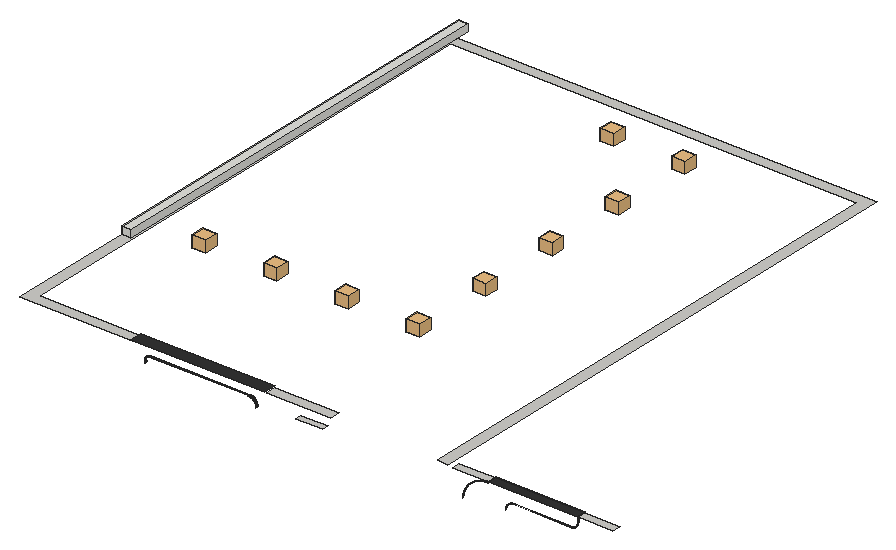
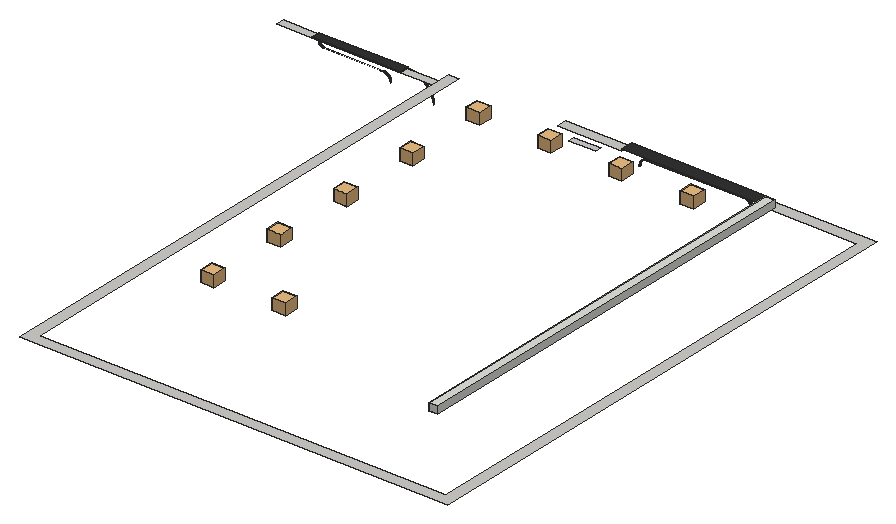
# SketchUp Ruby script. Lengths in inches.
U = 1.inch
M = Sketchup.active_model
def pt(a) = Geom::Point3d.new(a.map { |v| v * U })
def face(e, loops, mat)
  f = e.add_face(loops[0].map { |a| pt(a) })
  loops[1..].each { |l| e.add_face(l.map { |a| pt(a) }).erase! }
  f.material = f.back_material = mat if mat
  f
end
# faces: each face lists its corners as indices into pts; further lists are holes
def faces(e, pts, list, mat = nil) = list.each { |f| face(e, (f[0].is_a?(Array) ? f : [f]).map { |l| l.map { |i| pts[i] } }, mat) }
# xy, xz, yz: faces in a plane at the given z, y or x. An outline is a flat list of corners, or four numbers for a rectangle; further outlines are holes
def ring(l) = l.size == 4 ? [[l[0], l[1]], [l[2], l[1]], [l[2], l[3]], [l[0], l[3]]] : l.each_slice(2).to_a
def flat(e, list, mat, &to3) = list.each { |f| face(e, (f[0].is_a?(Array) ? f : [f]).map { |l| ring(l).map { |u, v| to3.(u, v) } }, mat) }
def xy(e, z, list, mat = nil) = flat(e, list, mat) { |x, y| [x, y, z] }
def xz(e, y, list, mat = nil) = flat(e, list, mat) { |x, z| [x, y, z] }
def yz(e, x, list, mat = nil) = flat(e, list, mat) { |y, z| [x, y, z] }
def lines(e, pts, list) = list.each { |a, b| e.add_line(pt(pts[a]), pt(pts[b])) }
# prism: a flat outline (further loops are holes) pulled along v
def prism(e, loops, v, mat = nil)
  f = face(e, loops, mat); d = Geom::Vector3d.new(v.map { |x| x * U })
  f.pushpull(f.normal.samedirection?(d) ? d.length : -d.length)
end
def box(e, o, s, mat = nil) = prism(e, [[o, [o[0] + s[0], o[1], o[2]], [o[0] + s[0], o[1] + s[1], o[2]], [o[0], o[1] + s[1], o[2]]]], [0, 0, s[2]], mat)
def at(x, y, z, deg = 0) = Geom::Transformation.translation(pt([x, y, z])) * Geom::Transformation.rotation(ORIGIN, Z_AXIS, deg.degrees)
def axes(o, x, y, z) = Geom::Transformation.new([*x, 0, *y, 0, *z, 0, *pt(o).to_a, 1])
def part(name) = M.definitions.add(name)
# library, detail: a bought-in or finely detailed component or shape, given as its bounding box
def library(name, o, s) = part(name).tap { |d| box(d.entities, o, s) }
def detail(e, o, s) = box(e.add_group.entities, o, s)
def put(e, d, t, mat = nil) = e.add_instance(d, t).tap { |i| i.material = mat if mat }
def group(e, t, mat = nil) = e.add_group.tap { |g| g.transformation = t; g.material = mat if mat }.entities
root = M.entities
M.materials.add("[Granite Dark Gray]").color = [51, 50, 50]
M.materials.add("[Stone Sandstone Ashlar Light]").color = [206, 205, 201]
c1 = library("6",[-5.64,-5.64,-12.71],[15.28,15.28,12.71])
xy(root,52.99,[[548.53,53,548.6875,54]],"[Granite Dark Gray]")
xy(root,53,[[548.84,53,549,54],[549,53,615,54],[615,53,615.12,54],[615.12,53,615.24,54]],"[Granite Dark Gray]")
xy(root,57,[[309,48,339,55]],"[Stone Sandstone Ashlar Light]")
xy(root,62.99,[[257.3125,46,257.47,48]],"[Granite Dark Gray]")
xy(root,63,[[146,46,257,48],[257,46,257.16,48]],"[Granite Dark Gray]")
xy(root,65,[[520.54,53,521,54]],"[Granite Dark Gray]")
xy(root,65,[[480,54,521,63],[621,54,660,63]],"[Stone Sandstone Ashlar Light]")
xy(root,66,[[521,53,621,63]],"[Granite Dark Gray]")
xy(root,71,[[0,48,126,48,126,60,12,60,12,636,468,636,468,48,480,48,480,648,0,648],[276,48,348,60]],"[Stone Sandstone Ashlar Light]")
xy(root,73,[[126,46,276,60]],"[Granite Dark Gray]")
xz(root,63,[[521,65,621,66]],"[Granite Dark Gray]")
yz(root,141.17,[[46,57.16,48,57.29],[46,57.29,48,57.42],[46,57.42,48,57.56]],"[Granite Dark Gray]")
yz(root,265.99,[[46,54.3125,48,54.47]],"[Granite Dark Gray]")
yz(root,266,[[46,54,48,54.16]],"[Granite Dark Gray]")
yz(root,521,[[53,65,63,66]],"[Granite Dark Gray]")
yz(root,540,[[53,44,54,44.16]],"[Granite Dark Gray]")
yz(root,540.01,[[53,44.3125,54,44.47]],"[Granite Dark Gray]")
yz(root,621,[[53,58.76,54,58.88],[53,58.88,54,59],[53,59,54,59,54,65,63,65,63,66,53,66]],"[Granite Dark Gray]")
p = [[491.79,54,39.66],[491.73,54,39.2],[491.73,53,39.2],[491.79,53,39.66],[491.86,54,40.11],[491.86,53,40.11],
  [491.9375,54,40.57],[491.9375,53,40.57],[492.02,54,41.03],[492.02,53,41.03],[492.11,54,41.48],[492.11,53,41.48],
  [492.21,54,41.94],[492.21,53,41.94],[492.32,54,42.39],[492.32,53,42.39],[492.43,54,42.84],[492.43,53,42.84],
  [492.55,54,43.28],[492.55,53,43.28],[492.67,54,43.73],[492.67,53,43.73],[492.8,54,44.17],[492.8,53,44.17],
  [492.94,54,44.62],[492.94,53,44.62],[540,54,44.16],[540.01,54,44.3125],[540.01,53,44.3125],[540,53,44.16],
  [540.01,54,44.47],[540.02,54,44.63],[540.02,53,44.63],[540.01,53,44.47],[493.09,54,45.06],[493.09,53,45.06],
  [540.03,54,44.78],[540.03,53,44.78],[540.05,54,44.94],[540.05,53,44.94],[540.07,54,45.1],[540.07,53,45.1],
  [493.24,54,45.49],[493.24,53,45.49],[540.09,54,45.25],[540.09,53,45.25],[540.11,54,45.41],[540.11,53,45.41],
  [540.14,54,45.5625],[540.14,53,45.5625],[493.4,54,45.93],[493.4,53,45.93],[540.17,54,45.72],[540.17,53,45.72],
  [540.2,54,45.87],[540.2,53,45.87],[493.57,54,46.36],[493.57,53,46.36],[540.23,54,46.02],[540.23,53,46.02],
  [540.27,54,46.18],[540.27,53,46.18],[540.31,54,46.33],[540.31,53,46.33],[540.35,54,46.48],[540.35,53,46.48],
  [493.75,54,46.79],[493.75,53,46.79],[540.39,54,46.63],[540.39,53,46.63],[540.44,54,46.78],[540.44,53,46.78],
  [493.93,54,47.22],[493.93,53,47.22],[540.49,54,46.93],[540.49,53,46.93],[540.54,54,47.08],[540.54,53,47.08],
  [540.6,54,47.23],[540.6,53,47.23],[494.11,54,47.64],[494.11,53,47.64],[540.66,54,47.37],[540.66,53,47.37],
  [540.72,54,47.52],[540.72,53,47.52],[540.78,54,47.66],[540.78,53,47.66],[494.31,54,48.06],[494.31,53,48.06],
  [540.84,54,47.8],[540.84,53,47.8],[540.91,54,47.95],[540.91,53,47.95],[540.98,54,48.09],[540.98,53,48.09],
  [494.51,54,48.48],[494.51,53,48.48],[541.05,54,48.23],[541.05,53,48.23],[541.13,54,48.36],[541.13,53,48.36],
  [541.21,54,48.5],[541.21,53,48.5],[494.72,54,48.89],[494.72,53,48.89],[541.29,54,48.64],[541.29,53,48.64],
  [541.37,54,48.77],[541.37,53,48.77],[541.45,54,48.9],[541.45,53,48.9],[494.93,54,49.3],[494.93,53,49.3],
  [541.54,54,49.03],[541.54,53,49.03],[541.63,54,49.16],[541.63,53,49.16],[541.72,54,49.29],[541.72,53,49.29],
  [495.15,54,49.71],[495.15,53,49.71],[541.8125,54,49.42],[541.8125,53,49.42],[541.91,54,49.54],[541.91,53,49.54],
  [542.01,54,49.66],[542.01,53,49.66],[495.375,54,50.12],[495.375,53,50.12],[542.11,54,49.79],[542.11,53,49.79],
  [542.21,54,49.9],[542.21,53,49.9],[542.3125,54,50.02],[542.3125,53,50.02],[542.42,54,50.14],[542.42,53,50.14],
  [495.61,54,50.52],[495.61,53,50.52],[542.53,54,50.25],[542.53,53,50.25],[542.64,54,50.36],[542.64,53,50.36],
  [542.75,54,50.47],[542.75,53,50.47],[495.85,54,50.91],[495.85,53,50.91],[542.86,54,50.58],[542.86,53,50.58],
  [542.98,54,50.6875],[542.98,53,50.6875],[543.1,54,50.79],[543.1,53,50.79],[543.21,54,50.89],[543.21,53,50.89],
  [496.09,54,51.31],[496.09,53,51.31],[543.34,54,50.99],[543.34,53,50.99],[543.46,54,51.09],[543.46,53,51.09],
  [543.58,54,51.1875],[543.58,53,51.1875],[543.71,54,51.28],[543.71,53,51.28],[496.34,54,51.7],[496.34,53,51.7],
  [543.84,54,51.37],[543.84,53,51.37],[543.97,54,51.46],[543.97,53,51.46],[544.1,54,51.55],[544.1,53,51.55],
  [544.23,54,51.63],[544.23,53,51.63],[544.36,54,51.71],[544.36,53,51.71],[496.6,54,52.08],[496.6,53,52.08],
  [544.5,54,51.79],[544.5,53,51.79],[544.64,54,51.87],[544.64,53,51.87],[544.77,54,51.95],[544.77,53,51.95],
  [544.91,54,52.02],[544.91,53,52.02],[545.05,54,52.09],[545.05,53,52.09],[496.86,54,52.46],[496.86,53,52.46],
  [545.2,54,52.16],[545.2,53,52.16],[545.34,54,52.22],[545.34,53,52.22],[545.48,54,52.28],[545.48,53,52.28],
  [545.63,54,52.34],[545.63,53,52.34],[545.77,54,52.4],[545.77,53,52.4],[545.92,54,52.46],[545.92,53,52.46],
  [497.13,54,52.84],[497.13,53,52.84],[546.07,54,52.51],[546.07,53,52.51],[546.22,54,52.56],[546.22,53,52.56],
  [546.37,54,52.61],[546.37,53,52.61],[546.52,54,52.65],[546.52,53,52.65],[546.67,54,52.69],[546.67,53,52.69],
  [546.82,54,52.73],[546.82,53,52.73],[546.98,54,52.77],[546.98,53,52.77],[497.41,54,53.21],[497.41,53,53.21],
  [547.13,54,52.8],[547.13,53,52.8],[547.28,54,52.83],[547.28,53,52.83],[547.4375,54,52.86],[547.4375,53,52.86],
  [547.59,54,52.89],[547.59,53,52.89],[547.75,54,52.91],[547.75,53,52.91],[547.9,54,52.93],[547.9,53,52.93],
  [548.06,54,52.95],[548.06,53,52.95],[548.22,54,52.97],[548.22,53,52.97],[548.37,54,52.98],[548.37,53,52.98],
  [548.53,54,52.99],[548.53,53,52.99],[548.6875,54,52.99],[548.84,54,53],[548.84,53,53],[548.6875,53,52.99],
  [615.24,54,53],[615.35,54,53.01],[615.35,53,53.01],[615.24,53,53],[615.47,54,53.02],[615.47,53,53.02],
  [615.59,54,53.03],[615.59,53,53.03],[615.71,54,53.04],[615.71,53,53.04],[615.82,54,53.06],[615.82,53,53.06],
  [615.9375,54,53.07],[615.9375,53,53.07],[616.05,54,53.09],[616.05,53,53.09],[616.17,54,53.12],[616.17,53,53.12],
  [616.29,54,53.14],[616.29,53,53.14],[616.4,54,53.17],[616.4,53,53.17],[497.69,54,53.58],[497.69,53,53.58],
  [616.51,54,53.19],[616.51,53,53.19],[616.63,54,53.23],[616.63,53,53.23],[616.74,54,53.26],[616.74,53,53.26],
  [616.85,54,53.29],[616.85,53,53.29],[616.97,54,53.33],[616.97,53,53.33],[617.08,54,53.37],[617.08,53,53.37],
  [617.1875,54,53.41],[617.1875,53,53.41],[617.3,54,53.46],[617.3,53,53.46],[617.4,54,53.5],[617.4,53,53.5],
  [617.51,54,53.55],[617.51,53,53.55],[497.98,54,53.94],[497.98,53,53.94],[617.62,54,53.6],[617.62,53,53.6],
  [617.72,54,53.65],[617.72,53,53.65],[617.83,54,53.71],[617.83,53,53.71],[617.93,54,53.77],[617.93,53,53.77],
  [618.03,54,53.82],[618.03,53,53.82],[618.13,54,53.88],[618.13,53,53.88],[498.27,54,54.3],[498.27,53,54.3],
  [618.23,54,53.95],[618.23,53,53.95],[618.33,54,54.01],[618.33,53,54.01],[618.43,54,54.08],[618.43,53,54.08],
  [618.53,54,54.15],[618.53,53,54.15],[618.62,54,54.22],[618.62,53,54.22],[266,46,54.16],[265.99,46,54.3125],
  [265.99,48,54.3125],[266,48,54.16],[618.71,54,54.29],[618.71,53,54.29],[498.57,54,54.66],[498.57,53,54.66],
  [618.81,54,54.36],[618.81,53,54.36],[618.9,54,54.4375],[618.9,53,54.4375],[618.99,54,54.51],[618.99,53,54.51],
  [265.99,46,54.47],[265.98,46,54.63],[265.98,48,54.63],[265.99,48,54.47],[619.07,54,54.59],[619.07,53,54.59],
  [265.97,46,54.78],[265.97,48,54.78],[619.16,54,54.67],[619.16,53,54.67],[498.87,54,55.01],[498.87,53,55.01],
  [619.24,54,54.76],[619.24,53,54.76],[265.95,46,54.94],[265.95,48,54.94],[619.33,54,54.84],[619.33,53,54.84],
  [619.41,54,54.93],[619.41,53,54.93],[265.93,46,55.1],[265.93,48,55.1],[619.49,54,55.01],[619.49,53,55.01],
  [141.64,46,55.12],[141.69,46,55],[141.69,48,55],[141.64,48,55.12],[499.18,54,55.35],[499.18,53,55.35],
  [619.5625,54,55.1],[619.5625,53,55.1],[141.59,46,55.24],[141.59,48,55.24],[265.91,46,55.25],[265.91,48,55.25],
  [619.64,54,55.19],[619.64,53,55.19],[141.54,46,55.36],[141.54,48,55.36],[619.71,54,55.29],[619.71,53,55.29],
  [265.89,46,55.41],[265.89,48,55.41],[619.78,54,55.38],[619.78,53,55.38],[141.49,46,55.49],[141.49,48,55.49],
  [265.86,46,55.5625],[265.86,48,55.5625],[499.5,54,55.69],[499.5,53,55.69],[619.85,54,55.47],[619.85,53,55.47],
  [141.45,46,55.61],[141.45,48,55.61],[619.92,54,55.57],[619.92,53,55.57],[141.41,46,55.74],[141.41,48,55.74],
  [265.83,46,55.72],[265.83,48,55.72],[619.99,54,55.67],[619.99,53,55.67],[141.375,46,55.86],[141.375,48,55.86],
  [265.8,46,55.87],[265.8,48,55.87],[499.82,54,56.03],[499.82,53,56.03],[620.05,54,55.77],[620.05,53,55.77],
  [620.12,54,55.87],[620.12,53,55.87],[141.34,46,55.99],[141.34,48,55.99],[265.77,46,56.02],[265.77,48,56.02],
  [620.18,54,55.97],[620.18,53,55.97],[141.3125,46,56.12],[141.3125,48,56.12],[265.73,46,56.18],[265.73,48,56.18],
  [500.14,54,56.36],[500.14,53,56.36],[620.23,54,56.07],[620.23,53,56.07],[141.28,46,56.25],[141.28,48,56.25],
  [620.29,54,56.17],[620.29,53,56.17],[141.26,46,56.38],[141.26,48,56.38],[265.69,46,56.33],[265.69,48,56.33],
  [620.35,54,56.28],[620.35,53,56.28],[265.65,46,56.48],[265.65,48,56.48],[620.4,54,56.38],[620.4,53,56.38],
  [141.24,46,56.51],[141.24,48,56.51],[500.47,54,56.68],[500.47,53,56.68],[620.45,54,56.49],[620.45,53,56.49],
  [141.22,46,56.64],[141.22,48,56.64],[265.61,46,56.63],[265.61,48,56.63],[620.5,54,56.6],[620.5,53,56.6],
  [141.2,46,56.77],[141.2,48,56.77],[265.56,46,56.78],[265.56,48,56.78],[620.54,54,56.7],[620.54,53,56.7],
  [500.81,54,57],[500.81,53,57],[620.59,54,56.8125],[620.59,53,56.8125],[141.19,46,56.9],[141.19,48,56.9],
  [265.51,46,56.93],[265.51,48,56.93],[620.63,54,56.92],[620.63,53,56.92],[141.18,46,57.03],[141.18,48,57.03],
  [265.46,46,57.08],[265.46,48,57.08],[620.67,54,57.03],[620.67,53,57.03],[141.17,46,57.16],[141.17,48,57.16],
  [501.15,54,57.32],[501.15,53,57.32],[620.71,54,57.15],[620.71,53,57.15],[265.4,46,57.23],[265.4,48,57.23],
  [620.74,54,57.26],[620.74,53,57.26],[265.34,46,57.37],[265.34,48,57.37],[501.49,54,57.63],[501.49,53,57.63],
  [620.77,54,57.37],[620.77,53,57.37],[265.28,46,57.52],[265.28,48,57.52],[620.81,54,57.49],[620.81,53,57.49],
  [265.22,46,57.66],[265.22,48,57.66],[620.83,54,57.6],[620.83,53,57.6],[141.18,46,57.6875],[141.17,46,57.56],
  [141.17,48,57.56],[141.18,48,57.6875],[501.84,54,57.93],[501.84,53,57.93],[620.86,54,57.71],[620.86,53,57.71],
  [141.1875,46,57.82],[141.1875,48,57.82],[265.16,46,57.8],[265.16,48,57.8],[620.88,54,57.83],[620.88,53,57.83],
  [141.2,46,57.95],[141.2,48,57.95],[265.09,46,57.95],[265.09,48,57.95],[620.91,54,57.95],[620.91,53,57.95],
  [265.02,46,58.09],[265.02,48,58.09],[502.2,54,58.23],[502.2,53,58.23],[620.93,54,58.0625],[620.93,53,58.0625],
  [141.21,46,58.08],[141.21,48,58.08],[141.23,46,58.21],[141.23,48,58.21],[264.95,46,58.23],[264.95,48,58.23],
  [620.94,54,58.18],[620.94,53,58.18],[141.25,46,58.34],[141.25,48,58.34],[264.87,46,58.36],[264.87,48,58.36],
  [502.56,54,58.52],[502.56,53,58.52],[620.96,54,58.29],[620.96,53,58.29],[141.27,46,58.47],[141.27,48,58.47],
  [620.97,54,58.41],[620.97,53,58.41],[264.79,46,58.5],[264.79,48,58.5],[620.98,54,58.53],[620.98,53,58.53],
  [141.3,46,58.6],[141.3,48,58.6],[264.71,46,58.64],[264.71,48,58.64],[502.92,54,58.81],[502.92,53,58.81],
  [620.99,54,58.65],[620.99,53,58.65],[141.33,46,58.73],[141.33,48,58.73],[264.63,46,58.77],[264.63,48,58.77],
  [621,54,58.76],[621,53,58.76],[141.36,46,58.86],[141.36,48,58.86],[264.55,46,58.9],[264.55,48,58.9],
  [503.29,54,59.09],[503.29,53,59.09],[141.4,46,58.98],[141.4,48,58.98],[264.46,46,59.03],[264.46,48,59.03],
  [141.4375,46,59.11],[141.4375,48,59.11],[264.37,46,59.16],[264.37,48,59.16],[141.48,46,59.23],[141.48,48,59.23],
  [503.66,54,59.37],[503.66,53,59.37],[141.52,46,59.36],[141.52,48,59.36],[264.28,46,59.29],[264.28,48,59.29],
  [264.1875,46,59.42],[264.1875,48,59.42],[141.57,46,59.48],[141.57,48,59.48],[264.09,46,59.54],[264.09,48,59.54],
  [504.04,54,59.64],[504.04,53,59.64],[141.62,46,59.6],[141.62,48,59.6],[263.99,46,59.66],[263.99,48,59.66],
  [141.67,46,59.72],[141.67,48,59.72],[504.42,54,59.9],[504.42,53,59.9],[141.73,46,59.84],[141.73,48,59.84],
  [263.89,46,59.79],[263.89,48,59.79],[141.79,46,59.96],[141.79,48,59.96],[263.79,46,59.9],[263.79,48,59.9],
  [263.6875,46,60.02],[263.6875,48,60.02],[504.8,54,60.16],[504.8,53,60.16],[141.85,46,60.08],[141.85,48,60.08],
  [263.58,46,60.14],[263.58,48,60.14],[141.91,46,60.19],[141.91,48,60.19],[263.47,46,60.25],[263.47,48,60.25],
  [141.98,46,60.3],[141.98,48,60.3],[505.19,54,60.41],[505.19,53,60.41],[142.05,46,60.42],[142.05,48,60.42],
  [263.36,46,60.36],[263.36,48,60.36],[142.12,46,60.53],[142.12,48,60.53],[263.25,46,60.47],[263.25,48,60.47],
  [505.59,54,60.65],[505.59,53,60.65],[142.19,46,60.64],[142.19,48,60.64],[263.14,46,60.58],[263.14,48,60.58],
  [142.27,46,60.74],[142.27,48,60.74],[263.02,46,60.6875],[263.02,48,60.6875],[142.35,46,60.85],[142.35,48,60.85],
  [262.9,46,60.79],[262.9,48,60.79],[505.98,54,60.89],[505.98,53,60.89],[142.43,46,60.95],[142.43,48,60.95],
  [262.79,46,60.89],[262.79,48,60.89],[262.66,46,60.99],[262.66,48,60.99],[506.38,54,61.125],[506.38,53,61.125],
  [142.51,46,61.05],[142.51,48,61.05],[262.54,46,61.09],[262.54,48,61.09],[142.6,46,61.15],[142.6,48,61.15],
  [262.42,46,61.1875],[262.42,48,61.1875],[506.79,54,61.35],[506.79,53,61.35],[142.6875,46,61.25],[142.6875,48,61.25],
  [142.78,46,61.34],[142.78,48,61.34],[262.29,46,61.28],[262.29,48,61.28],[142.87,46,61.4375],[142.87,48,61.4375],
  [262.16,46,61.37],[262.16,48,61.37],[142.97,46,61.53],[142.97,48,61.53],[262.03,46,61.46],[262.03,48,61.46],
  [507.2,54,61.57],[507.2,53,61.57],[143.06,46,61.62],[143.06,48,61.62],[261.9,46,61.55],[261.77,46,61.63],
  [261.77,48,61.63],[261.9,48,61.55],[143.16,46,61.7],[143.16,48,61.7],[261.64,46,61.71],[261.64,48,61.71],
  [507.61,54,61.78],[507.61,53,61.78],[143.26,46,61.79],[143.26,48,61.79],[261.5,46,61.79],[261.5,48,61.79],
  [143.37,46,61.87],[143.37,48,61.87],[261.36,46,61.87],[261.36,48,61.87],[508.02,54,61.99],[508.02,53,61.99],
  [143.47,46,61.95],[143.47,48,61.95],[261.23,46,61.95],[261.09,46,62.02],[261.09,48,62.02],[261.23,48,61.95],
  [143.58,46,62.03],[143.58,48,62.03],[143.6875,46,62.1],[143.6875,48,62.1],[260.95,46,62.09],[260.95,48,62.09],
  [508.44,54,62.19],[508.44,53,62.19],[143.8,46,62.17],[143.8,48,62.17],[260.8,46,62.16],[260.8,48,62.16],
  [143.91,46,62.24],[143.91,48,62.24],[144.02,46,62.31],[144.02,48,62.31],[260.66,46,62.22],[260.52,46,62.28],
  [260.52,48,62.28],[260.66,48,62.22],[508.86,54,62.39],[508.86,53,62.39],[144.14,46,62.375],[144.14,48,62.375],
  [260.37,46,62.34],[260.23,46,62.4],[260.23,48,62.4],[260.37,48,62.34],[144.25,46,62.4375],[144.25,48,62.4375],
  [144.37,46,62.49],[144.37,48,62.49],[260.08,46,62.46],[260.08,48,62.46],[509.28,54,62.57],[509.28,53,62.57],
  [144.49,46,62.55],[144.49,48,62.55],[259.93,46,62.51],[259.78,46,62.56],[259.78,48,62.56],[259.93,48,62.51],
  [144.61,46,62.6],[144.61,48,62.6],[144.73,46,62.65],[144.73,48,62.65],[259.63,46,62.61],[259.48,46,62.65],
  [259.48,48,62.65],[259.63,48,62.61],[509.71,54,62.75],[509.71,53,62.75],[144.86,46,62.7],[144.86,48,62.7],
  [144.98,46,62.75],[144.98,48,62.75],[145.1,46,62.79],[145.1,48,62.79],[259.18,46,62.73],[259.02,46,62.77],
  [259.02,48,62.77],[259.18,48,62.73],[259.33,46,62.69],[259.33,48,62.69],[145.23,46,62.83],[145.23,48,62.83],
  [145.36,46,62.86],[145.36,48,62.86],[258.72,46,62.83],[258.5625,46,62.86],[258.5625,48,62.86],[258.72,48,62.83],
  [258.87,46,62.8],[258.87,48,62.8],[510.14,54,62.93],[510.14,53,62.93],[145.48,46,62.9],[145.48,48,62.9],
  [145.61,46,62.93],[145.61,48,62.93],[145.74,46,62.95],[145.74,48,62.95],[258.1,46,62.93],[257.94,46,62.95],
  [257.94,48,62.95],[258.1,48,62.93],[258.25,46,62.91],[258.25,48,62.91],[258.41,46,62.89],[258.41,48,62.89],
  [510.57,54,63.1],[510.57,53,63.1],[145.87,46,62.98],[145.87,48,62.98],[146,46,63],[146,48,63],
  [257.3125,46,62.99],[257.16,46,63],[257.16,48,63],[257.3125,48,62.99],[257.63,46,62.98],[257.47,46,62.99],
  [257.47,48,62.99],[257.63,48,62.98],[257.78,46,62.97],[257.78,48,62.97],[511.01,54,63.26],[511.01,53,63.26],
  [511.44,54,63.41],[511.44,53,63.41],[511.88,54,63.56],[511.88,53,63.56],[512.33,54,63.7],[512.33,53,63.7],
  [512.77,54,63.83],[512.77,53,63.83],[513.22,54,63.95],[513.22,53,63.95],[513.66,54,64.07],[513.66,53,64.07],
  [514.11,54,64.18],[514.11,53,64.18],[514.56,54,64.29],[514.56,53,64.29],[515.02,54,64.39],[515.02,53,64.39],
  [515.47,54,64.48],[515.47,53,64.48],[515.93,54,64.5625],[515.93,53,64.5625],[516.39,54,64.64],[516.39,53,64.64],
  [516.84,54,64.71],[516.84,53,64.71],[517.3,54,64.77],[517.3,53,64.77],[517.76,54,64.82],[517.76,53,64.82],
  [518.22,54,64.87],[518.22,53,64.87],[518.69,54,64.91],[518.69,53,64.91],[519.15,54,64.94],[519.15,53,64.94],
  [519.61,54,64.97],[519.61,53,64.97],[520.07,54,64.99],[520.07,53,64.99],[520.54,54,65],[520.54,53,65],
  [266,48,63],[257,48,63],[138,48,63],[138,46,63],[266,46,63],[266,48,54]]
faces(root,p,[[0,1,2,3],[4,0,3,5],[6,4,5,7],[8,6,7,9],[10,8,9,11],[12,10,11,13],[14,12,13,15],[16,14,15,17],
  [18,16,17,19],[20,18,19,21],[22,20,21,23],[24,22,23,25],[26,27,28,29],[30,31,32,33],[34,24,25,35],[31,36,37,32],
  [36,38,39,37],[38,40,41,39],[42,34,35,43],[40,44,45,41],[44,46,47,45],[46,48,49,47],[50,42,43,51],[48,52,53,49],
  [52,54,55,53],[56,50,51,57],[54,58,59,55],[58,60,61,59],[60,62,63,61],[62,64,65,63],[66,56,57,67],[64,68,69,65],
  [68,70,71,69],[72,66,67,73],[70,74,75,71],[74,76,77,75],[76,78,79,77],[80,72,73,81],[78,82,83,79],[82,84,85,83],
  [84,86,87,85],[88,80,81,89],[86,90,91,87],[90,92,93,91],[92,94,95,93],[96,88,89,97],[94,98,99,95],[98,100,101,99],
  [100,102,103,101],[104,96,97,105],[102,106,107,103],[106,108,109,107],[108,110,111,109],[112,104,105,113],[110,114,115,111],[114,116,117,115],
  [116,118,119,117],[120,112,113,121],[118,122,123,119],[122,124,125,123],[124,126,127,125],[128,120,121,129],[126,130,131,127],[130,132,133,131],
  [132,134,135,133],[134,136,137,135],[138,128,129,139],[136,140,141,137],[140,142,143,141],[142,144,145,143],[146,138,139,147],[144,148,149,145],
  [148,150,151,149],[150,152,153,151],[152,154,155,153],[156,146,147,157],[154,158,159,155],[158,160,161,159],[160,162,163,161],[162,164,165,163],
  [166,156,157,167],[164,168,169,165],[168,170,171,169],[170,172,173,171],[172,174,175,173],[174,176,177,175],[178,166,167,179],[176,180,181,177],
  [180,182,183,181],[182,184,185,183],[184,186,187,185],[186,188,189,187],[190,178,179,191],[188,192,193,189],[192,194,195,193],[194,196,197,195],
  [196,198,199,197],[198,200,201,199],[200,202,203,201],[204,190,191,205],[202,206,207,203],[206,208,209,207],[208,210,211,209],[210,212,213,211],
  [212,214,215,213],[214,216,217,215],[216,218,219,217],[220,204,205,221],[218,222,223,219],[222,224,225,223],[224,226,227,225],[226,228,229,227],
  [228,230,231,229],[230,232,233,231],[232,234,235,233],[234,236,237,235],[236,238,239,237],[238,240,241,239],[242,243,244,245],[246,247,248,249],
  [247,250,251,248],[250,252,253,251],[252,254,255,253],[254,256,257,255],[256,258,259,257],[258,260,261,259],[260,262,263,261],[262,264,265,263],
  [264,266,267,265],[268,220,221,269],[266,270,271,267],[270,272,273,271],[272,274,275,273],[274,276,277,275],[276,278,279,277],[278,280,281,279],
  [280,282,283,281],[282,284,285,283],[284,286,287,285],[286,288,289,287],[290,268,269,291],[288,292,293,289],[292,294,295,293],[294,296,297,295],
  [296,298,299,297],[298,300,301,299],[300,302,303,301],[304,290,291,305],[302,306,307,303],[306,308,309,307],[308,310,311,309],[310,312,313,311],
  [312,314,315,313],[316,317,318,319],[314,320,321,315],[322,304,305,323],[320,324,325,321],[324,326,327,325],[326,328,329,327],[330,331,332,333],
  [328,334,335,329],[331,336,337,332],[334,338,339,335],[340,322,323,341],[338,342,343,339],[336,344,345,337],[342,346,347,343],[346,348,349,347],
  [344,350,351,345],[348,352,353,349],[354,355,356,357],[358,340,341,359],[352,360,361,353],[362,354,357,363],[350,364,365,351],[360,366,367,361],
  [368,362,363,369],[366,370,371,367],[364,372,373,365],[370,374,375,371],[376,368,369,377],[372,378,379,373],[380,358,359,381],[374,382,383,375],
  [384,376,377,385],[382,386,387,383],[388,384,385,389],[378,390,391,379],[386,392,393,387],[394,388,389,395],[390,396,397,391],[398,380,381,399],
  [392,400,401,393],[400,402,403,401],[404,394,395,405],[396,406,407,397],[402,408,409,403],[410,404,405,411],[406,412,413,407],[414,398,399,415],
  [408,416,417,409],[418,410,411,419],[416,420,421,417],[422,418,419,423],[412,424,425,413],[420,426,427,421],[424,428,429,425],[426,430,431,427],
  [432,422,423,433],[434,414,415,435],[430,436,437,431],[438,432,433,439],[428,440,441,429],[436,442,443,437],[444,438,439,445],[440,446,447,441],
  [442,448,449,443],[450,434,435,451],[448,452,453,449],[454,444,445,455],[446,456,457,447],[452,458,459,453],[460,454,455,461],[456,462,463,457],
  [458,464,465,459],[466,460,461,467],[468,450,451,469],[464,470,471,465],[462,472,473,463],[470,474,475,471],[472,476,477,473],[478,468,469,479],
  [474,480,481,475],[476,482,483,477],[480,484,485,481],[482,486,487,483],[484,488,489,485],[490,491,492,493],[494,478,479,495],[488,496,497,489],
  [498,490,493,499],[486,500,501,487],[496,502,503,497],[504,498,499,505],[500,506,507,501],[502,508,509,503],[506,510,511,507],[512,494,495,513],
  [508,514,515,509],[516,504,505,517],[518,516,517,519],[510,520,521,511],[514,522,523,515],[524,518,519,525],[520,526,527,521],[528,512,513,529],
  [522,530,531,523],[532,524,525,533],[530,534,535,531],[526,536,537,527],[534,538,539,535],[540,532,533,541],[536,542,543,537],[544,528,529,545],
  [538,546,547,539],[548,540,541,549],[542,550,551,543],[546,552,553,547],[554,548,549,555],[550,556,557,551],[558,544,545,559],[560,554,555,561],
  [556,562,563,557],[564,560,561,565],[562,566,567,563],[568,564,565,569],[570,558,559,571],[572,568,569,573],[566,574,575,567],[574,576,577,575],
  [578,572,573,579],[576,580,581,577],[582,570,571,583],[584,578,579,585],[580,586,587,581],[588,584,585,589],[590,582,583,591],[592,588,589,593],
  [586,594,595,587],[596,592,593,597],[594,598,599,595],[598,600,601,599],[602,590,591,603],[604,596,597,605],[600,606,607,601],[608,604,605,609],
  [606,610,611,607],[612,608,609,613],[614,602,603,615],[616,612,613,617],[610,618,619,611],[620,616,617,621],[618,622,623,619],[624,614,615,625],
  [626,620,621,627],[622,628,629,623],[630,626,627,631],[628,632,633,629],[634,630,631,635],[632,636,637,633],[638,624,625,639],[640,634,635,641],
  [636,642,643,637],[642,644,645,643],[646,638,639,647],[648,640,641,649],[644,650,651,645],[652,648,649,653],[650,654,655,651],[656,646,647,657],
  [658,652,653,659],[660,658,659,661],[654,662,663,655],[664,660,661,665],[662,666,667,663],[668,664,665,669],[666,670,671,667],[672,656,657,673],
  [674,668,669,675],[676,677,678,679],[670,676,679,671],[680,674,675,681],[677,682,683,678],[684,672,673,685],[686,680,681,687],[682,688,689,683],
  [690,686,687,691],[688,692,693,689],[694,684,685,695],[696,690,691,697],[698,699,700,701],[692,698,701,693],[702,696,697,703],[704,702,703,705],
  [699,706,707,700],[708,694,695,709],[710,704,705,711],[706,712,713,707],[714,710,711,715],[716,714,715,717],[718,719,720,721],[712,718,721,713],
  [722,708,709,723],[724,716,717,725],[726,727,728,729],[719,726,729,720],[730,724,725,731],[732,730,731,733],[727,734,735,728],[736,722,723,737],
  [738,732,733,739],[740,741,742,743],[734,740,743,735],[744,738,739,745],[746,744,745,747],[748,749,750,751],[741,748,751,742],[752,736,737,753],
  [754,746,747,755],[756,754,755,757],[758,756,757,759],[760,761,762,763],[764,760,763,765],[749,764,765,750],[766,758,759,767],[768,766,767,769],
  [770,771,772,773],[774,770,773,775],[761,774,775,762],[776,752,753,777],[778,768,769,779],[780,778,779,781],[782,780,781,783],[784,785,786,787],
  [788,784,787,789],[790,788,789,791],[771,790,791,772],[792,776,777,793],[794,782,783,795],[796,794,795,797],[798,799,800,801],[802,803,804,805],
  [806,802,805,807],[785,806,807,786],[808,792,793,809],[810,808,809,811],[812,810,811,813],[814,812,813,815],[816,814,815,817],[818,816,817,819],
  [820,818,819,821],[822,820,821,823],[824,822,823,825],[826,824,825,827],[828,826,827,829],[830,828,829,831],[832,830,831,833],[834,832,833,835],
  [836,834,835,837],[838,836,837,839],[840,838,839,841],[842,840,841,843],[844,842,843,845],[846,844,845,847],[848,846,847,849],[850,848,849,851]],"[Granite Dark Gray]")
lines(root,p,[[852,853],[854,356],[855,854],[797,854],[856,852],[857,852]])
put(root,c1,at(358,433,128.5))
put(root,c1,at(358,247,128.5))
put(root,c1,at(358,340,128.5))
put(root,c1,at(198,154,128.5))
put(root,c1,at(358,154,128.5))
put(root,c1,at(278,154,128.5))
put(root,c1,at(118,154,128.5))
put(root,c1,at(358,526,128.5))
put(root,c1,at(278,526,128.5))
g1 = group(root,at(54,183,121.75))
box(g1,[0,-60,-2],[10,472,8])
